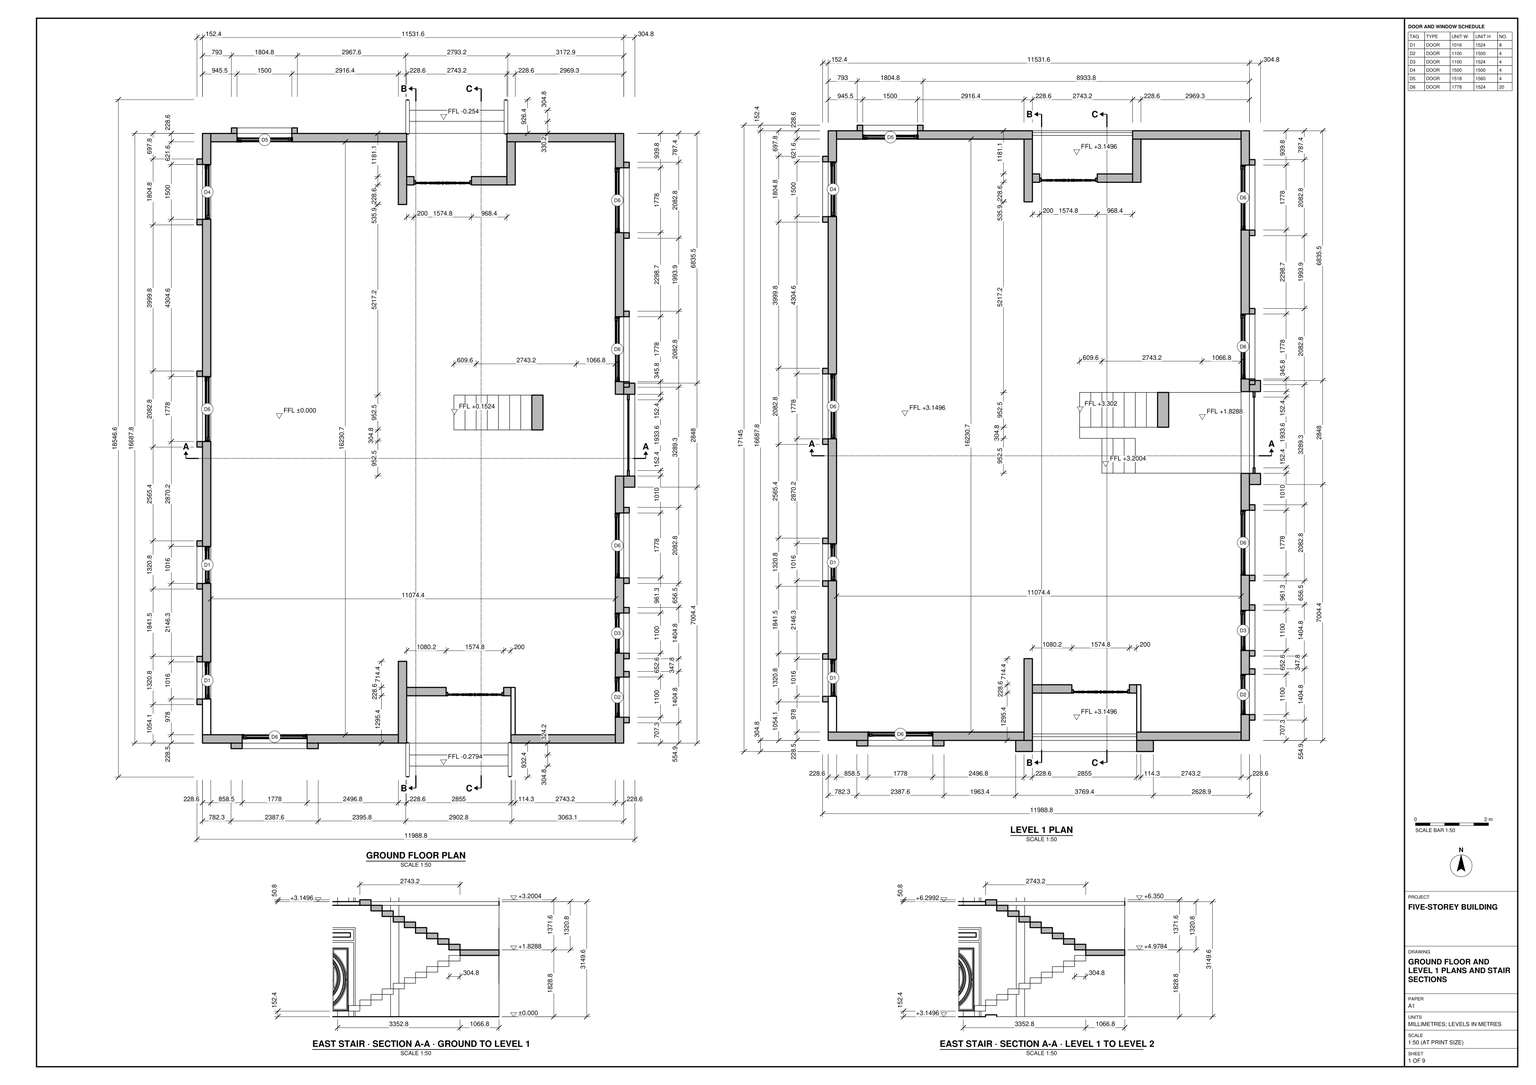
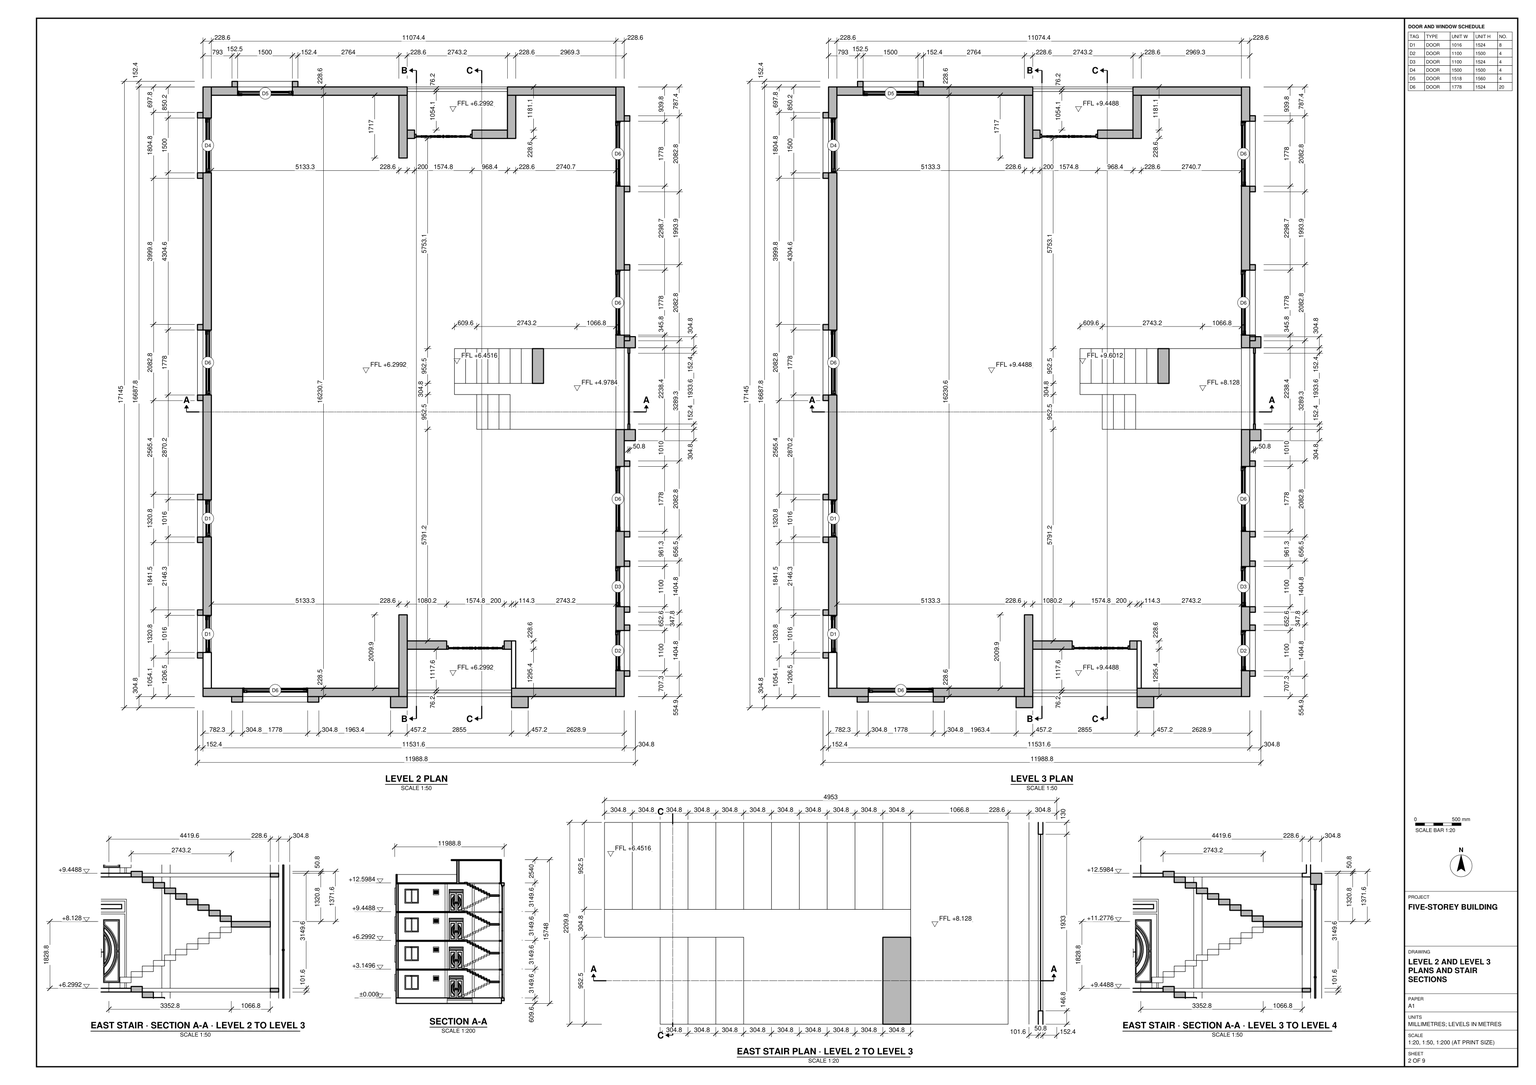
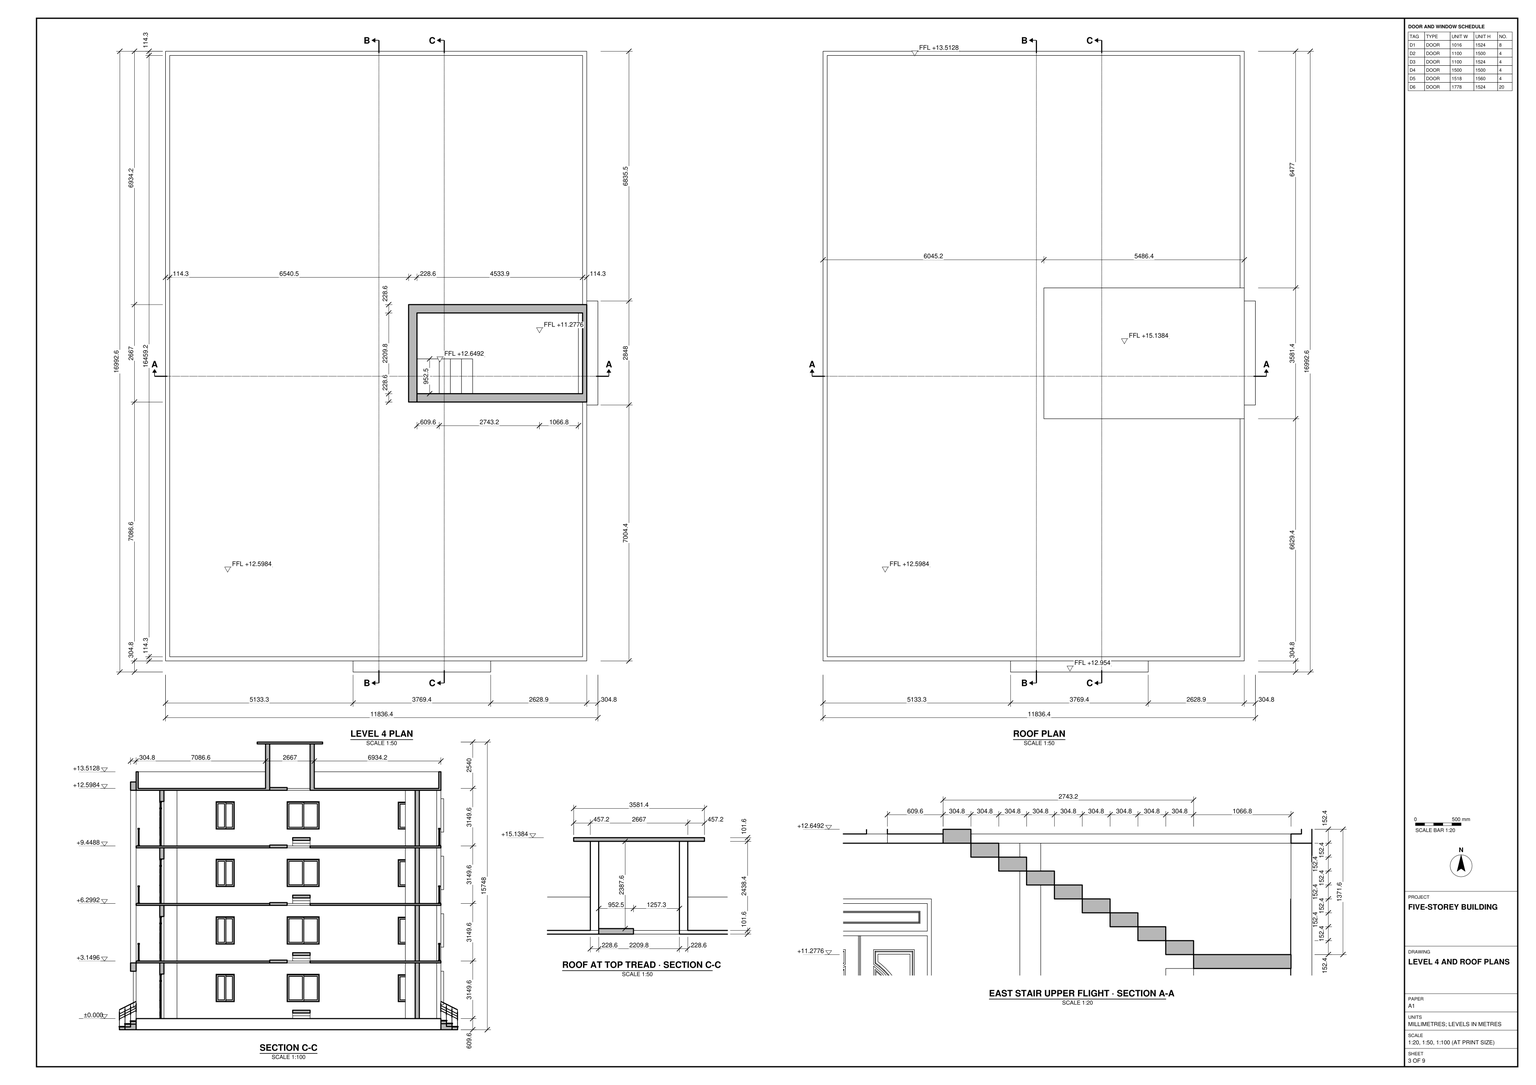
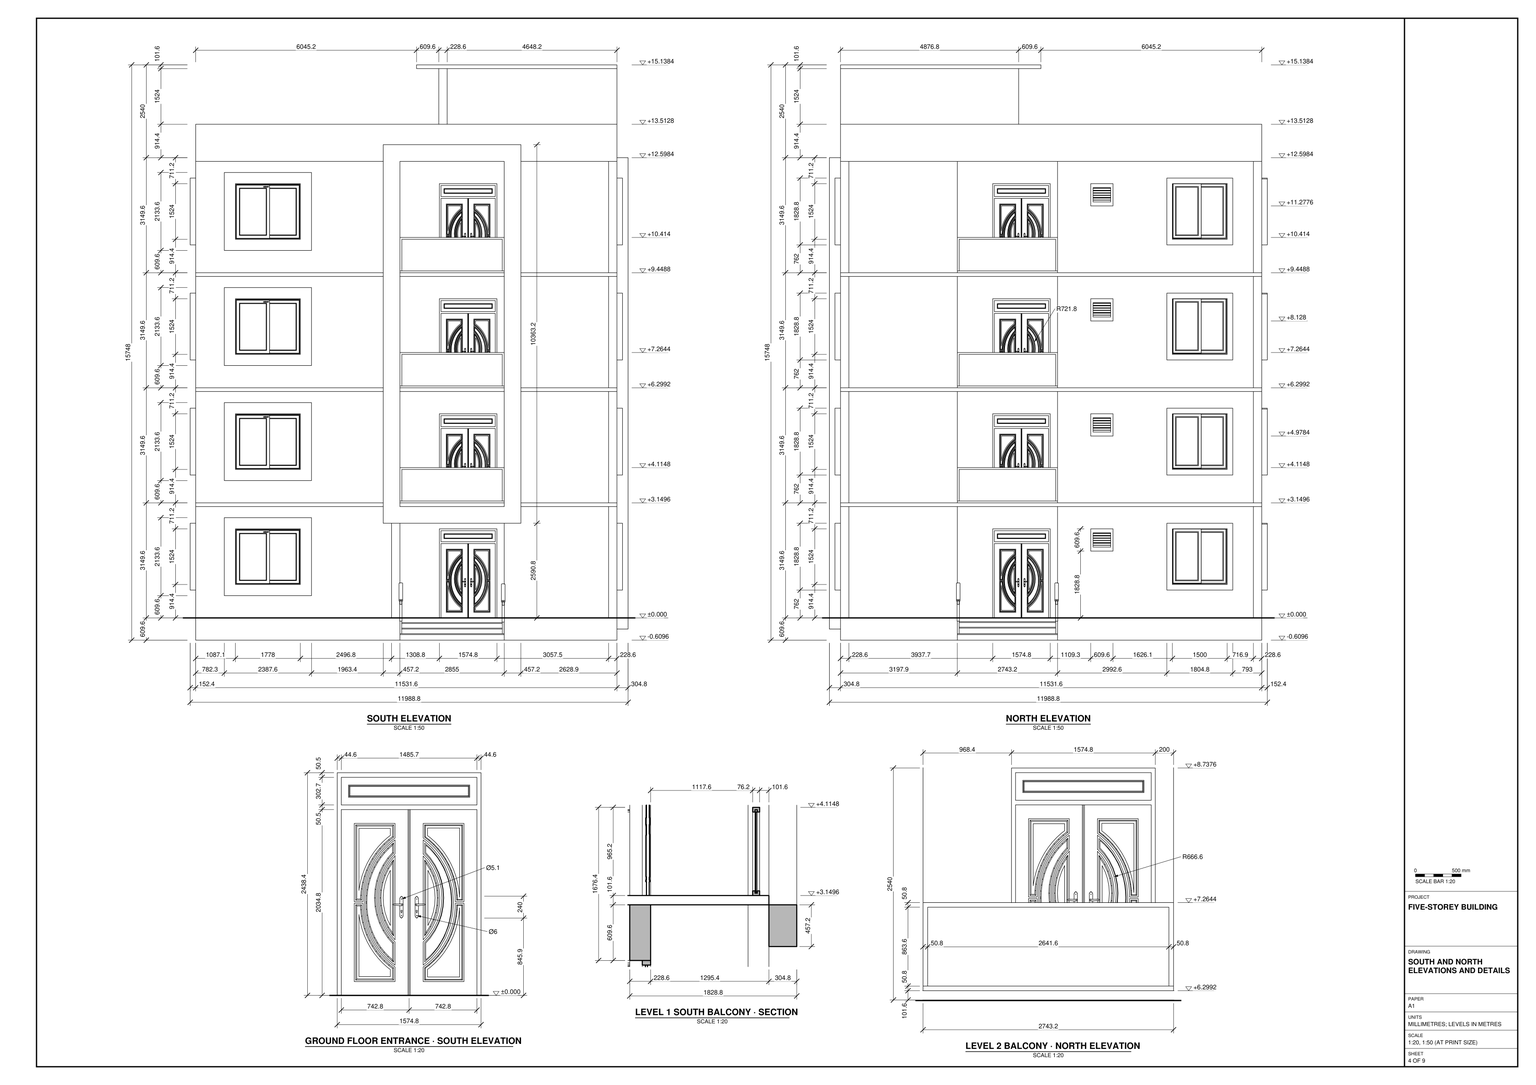
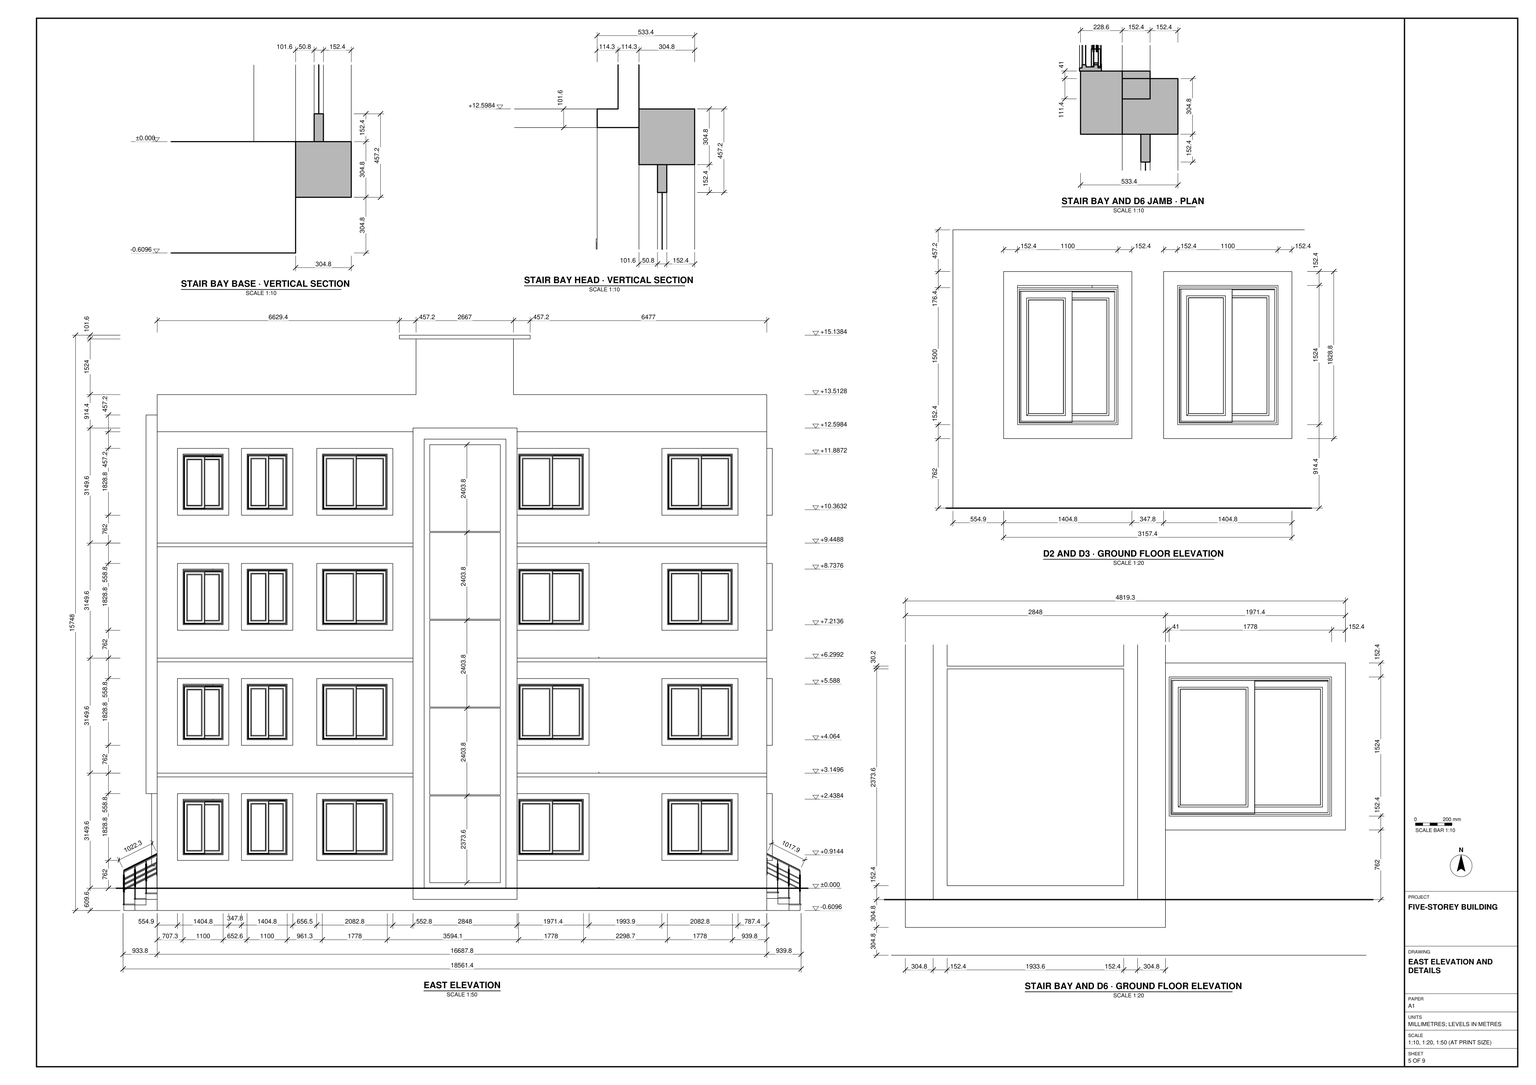
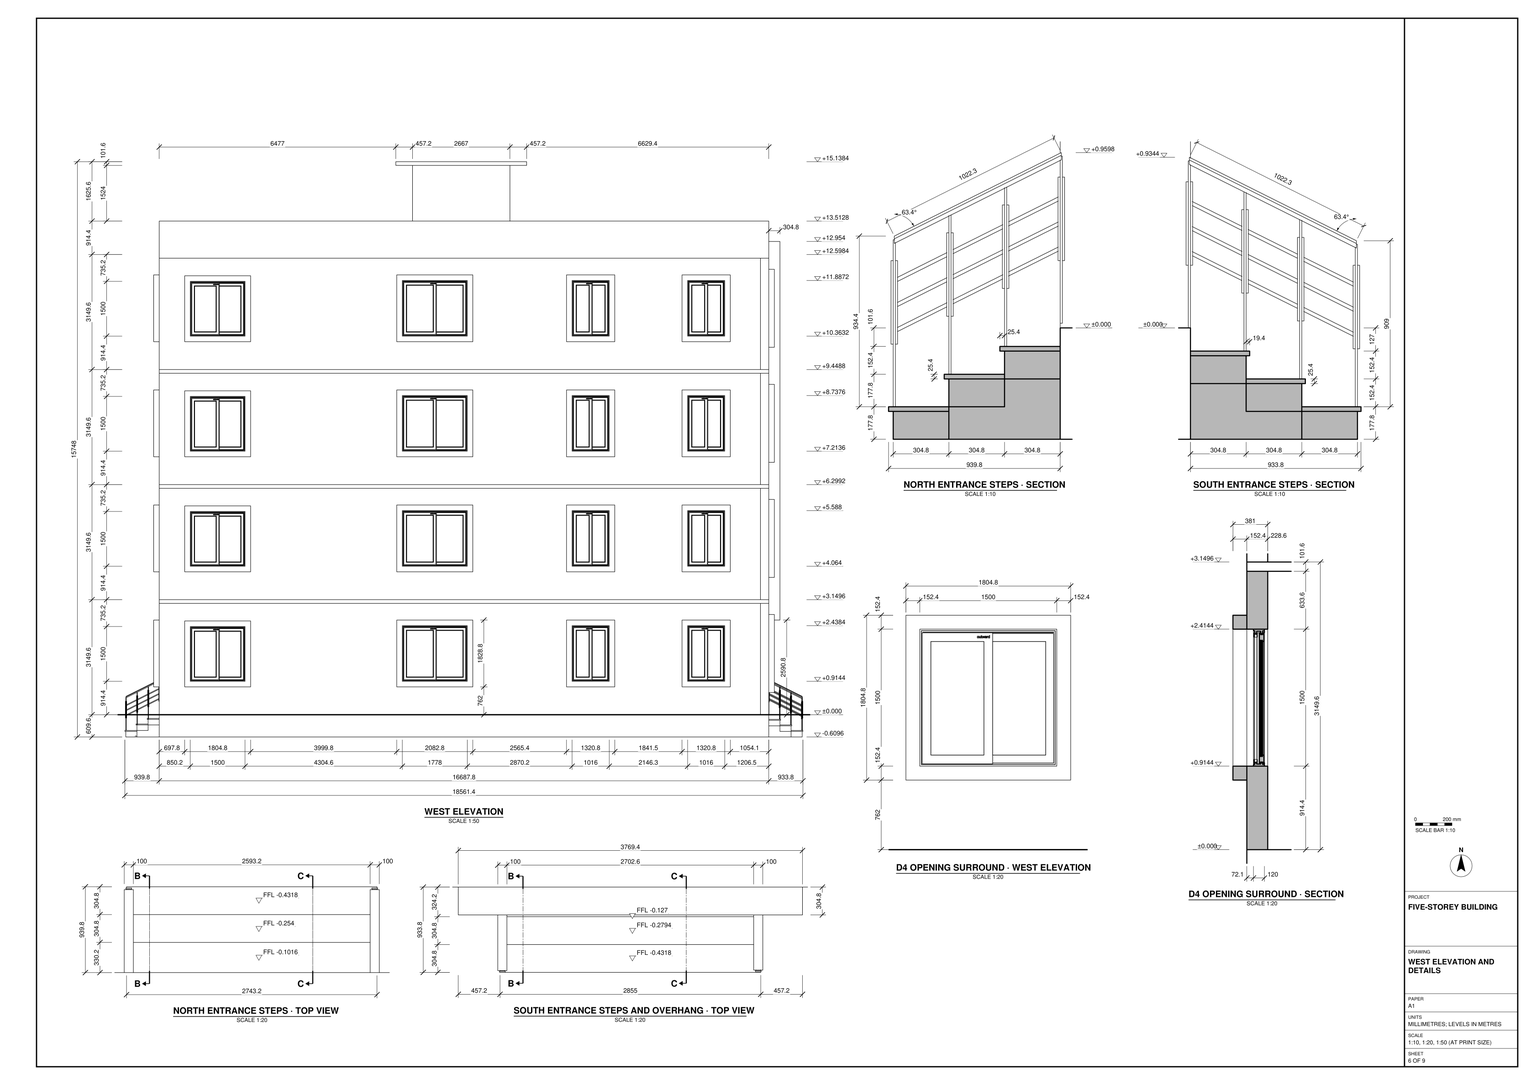
Use task_files/diagram_01.pdf to build the model in SketchUp. Work in millimetres. Set out the building with its short sides facing north and south. The overall extents are 11988.8 mm along X, 18561.4 mm along Y and 15748 mm from base to top. Use finished floor levels of 0 mm, +3149.6 mm, +6299.2 mm, +9448.8 mm and +12598.4 mm relative to the ground floor.

Build the base, floor slabs and perimeter walls, keeping the enclosed floors largely open as shown in plan. Follow the drawn wall thicknesses and reproduce the wall returns that form the recessed entrances at the north and south ends. Include the exterior approach steps and railings. Use the plans and schedule to size and place the doors and window units, retaining the frames and the vertical alignment of corresponding openings.

Use the stair sections to model the two returning flights on the east side, their intermediate landings and the openings through the slabs. At level 4, form the flat roof with its perimeter parapet and the raised enclosure over the stair. Keep shell elements and any furniture or joinery pieces in separate groups or components, and use components for repeated parts. Decor and loose items shown may be any suitable library components. Save one SketchUp model as output_files/five_storey_building_with_east_stair_and_roof_access.skp.

# SketchUp Ruby script. Lengths in millimetres.
U = 1.mm
M = Sketchup.active_model
def pt(a) = Geom::Point3d.new(a.map { |v| v * U })
def face(e, loops, mat)
  f = e.add_face(loops[0].map { |a| pt(a) })
  loops[1..].each { |l| e.add_face(l.map { |a| pt(a) }).erase! }
  f.material = f.back_material = mat if mat
  f
end
# faces: each face lists its corners as indices into pts; further lists are holes
def faces(e, pts, list, mat = nil) = list.each { |f| face(e, (f[0].is_a?(Array) ? f : [f]).map { |l| l.map { |i| pts[i] } }, mat) }
# xy, xz, yz: faces in a plane at the given z, y or x. An outline is a flat list of corners, or four numbers for a rectangle; further outlines are holes
def ring(l) = l.size == 4 ? [[l[0], l[1]], [l[2], l[1]], [l[2], l[3]], [l[0], l[3]]] : l.each_slice(2).to_a
def flat(e, list, mat, &to3) = list.each { |f| face(e, (f[0].is_a?(Array) ? f : [f]).map { |l| ring(l).map { |u, v| to3.(u, v) } }, mat) }
def xy(e, z, list, mat = nil) = flat(e, list, mat) { |x, y| [x, y, z] }
def xz(e, y, list, mat = nil) = flat(e, list, mat) { |x, z| [x, y, z] }
def yz(e, x, list, mat = nil) = flat(e, list, mat) { |y, z| [x, y, z] }
def lines(e, pts, list) = list.each { |a, b| e.add_line(pt(pts[a]), pt(pts[b])) }
# prism: a flat outline (further loops are holes) pulled along v
def prism(e, loops, v, mat = nil)
  f = face(e, loops, mat); d = Geom::Vector3d.new(v.map { |x| x * U })
  f.pushpull(f.normal.samedirection?(d) ? d.length : -d.length)
end
def box(e, o, s, mat = nil) = prism(e, [[o, [o[0] + s[0], o[1], o[2]], [o[0] + s[0], o[1] + s[1], o[2]], [o[0], o[1] + s[1], o[2]]]], [0, 0, s[2]], mat)
def at(x, y, z, deg = 0) = Geom::Transformation.translation(pt([x, y, z])) * Geom::Transformation.rotation(ORIGIN, Z_AXIS, deg.degrees)
def axes(o, x, y, z) = Geom::Transformation.new([*x, 0, *y, 0, *z, 0, *pt(o).to_a, 1])
def part(name) = M.definitions.add(name)
# library, detail: a bought-in or finely detailed component or shape, given as its bounding box
def library(name, o, s) = part(name).tap { |d| box(d.entities, o, s) }
def detail(e, o, s) = box(e.add_group.entities, o, s)
def put(e, d, t, mat = nil) = e.add_instance(d, t).tap { |i| i.material = mat if mat }
def group(e, t, mat = nil) = e.add_group.tap { |g| g.transformation = t; g.material = mat if mat }.entities
root = M.entities
M.materials.add("TEAKcrown-cut").color = [186, 122, 55]
M.materials.add("[Brick Colored Blue]").color = [144, 143, 146]
M.materials.add("[Brick Rough Dark]").color = [94, 77, 53]
M.materials.add("[Color M05]").color = [114, 114, 114]
M.materials.add("[Color M06]").color = [86, 86, 86]
M.materials.add("[Color M07]").color = [58, 58, 58]
M.materials.add("[Translucent Glass Gray]").color = [128, 128, 128]
M.materials["[Translucent Glass Gray]"].alpha = 0.5
M.materials.add("[Translucent Glass Sky Reflection]").color = [124, 138, 181]
M.materials["[Translucent Glass Sky Reflection]"].alpha = 0.5
M.materials.add("[Translucent_Glass_Gray]3").color = [255, 255, 255]
M.materials["[Translucent_Glass_Gray]3"].alpha = 0.5
c1 = part("Component\#10")
box(c1.entities,[0,0,0],[482.6,6.4,94],"[Translucent_Glass_Gray]3")
c2 = part("Ventilation_window")
g1 = group(c2.entities,at(-1953.5,162,0),"TEAKcrown-cut")
xy(g1,-43.2,[[0,0,609.6,76.2]])
xy(g1,63.5,[[63.5,0,546.1,76.2]])
xy(g1,444.5,[[63.5,0,546.1,76.2]])
xy(g1,551.2,[[0,0,609.6,76.2]])
xz(g1,0,[[[0,-43.2,609.6,551.2],[63.5,63.5,546.1,444.5]]],"TEAKcrown-cut")
xz(g1,76.2,[[[0,-43.2,609.6,551.2],[63.5,63.5,546.1,444.5]]])
yz(g1,0,[[0,-43.2,76.2,551.2]])
yz(g1,63.5,[[0,63.5,76.2,63.5,76.2,109.5,0,164.5],[76.2,109.5,76.2,444.5,0,444.5,0,164.5]])
yz(g1,546.1,[[0,63.5,76.2,444.5]])
yz(g1,609.6,[[0,-43.2,76.2,551.2]])
put(g1,c1,axes([63.5,79.8,303.2],[1,0,0],[0,0.58779,0.80902],[0,-0.80902,0.58779]))
put(g1,c1,axes([63.5,80.3,370.9],[1,0,0],[0,0.58779,0.80902],[0,-0.80902,0.58779]))
put(g1,c1,axes([63.5,76.2,109.5],[1,0,0],[0,0.58779,0.80902],[0,-0.80902,0.58779]))
put(g1,c1,axes([63.5,79.8,240.3],[1,0,0],[0,0.58779,0.80902],[0,-0.80902,0.58779]))
put(g1,c1,axes([63.5,76,179.9],[1,0,0],[0,0.58779,0.80902],[0,-0.80902,0.58779]))
c3 = library("AS-120-mm\#4",[0,0,0],[1016,120,1524])
c4 = library("AS-120-mm\#2",[0,0,0],[1500,120,1500])
c5 = library("AS-120-mm\#1",[0,0,0],[1518,120,1560])
c6 = library("AS-120-mm\#3",[0,0,0],[1778,120,1524])
c7 = library("AS-120-mm\#5",[0,0,0],[1778,120,1524])
c8 = library("AS-120-mm\#10",[0,0,0],[1778,120,1524])
c9 = library("AS-120-mm\#7",[0,0,0],[1100,120,1524])
c10 = library("AS-120-mm\#6",[0,0,0],[1100,120,1500])
c11 = library("AS-120-mm\#8",[0,0,0],[1778,120,1524])
c12 = library("AS-120-mm\#9",[0,0,0],[1778,120,1524])
c13 = part("Group\#4")
box(c13.entities,[0,0,0],[2969.3,228.6,3048])
c14 = part("Group\#14")
prism(c14.entities,[[[2743.2,228.6,0],[1774.8,228.6,0],[1774.8,228.6,2438.4],[200,228.6,2438.4],[200,228.6,0],[0,228.6,0],[0,228.6,3048],[2743.2,228.6,3048]]],[0,-228.6,0])
c15 = part("Group\#15")
box(c15.entities,[0,0,0],[228.6,1717,3048])
c16 = part("Group\#8")
box(c16.entities,[0,0,0],[304.8,952.5,152.4])
c17 = part("Group\#10")
box(c17.entities,[0,0,0],[228.6,2238.4,3048])
c18 = part("Group\#6")
box(c18.entities,[0,0,0],[2857.5,228.6,3048])
c19 = part("Group\#7")
box(c19.entities,[0,-1257.3,0],[1066.8,2209.8,152.4])
c20 = part("Group\#2")
prism(c20.entities,[[[228.6,0,0],[228.6,16459.2,0],[228.6,16459.2,3048],[228.6,0,3048]],[[228.6,9804.4,2438.4],[228.6,9804.4,914.4],[228.6,8026.4,914.4],[228.6,8026.4,2438.4]],[[228.6,14109,914.4],[228.6,14109,2414.4],[228.6,15609,2414.4],[228.6,15609,914.4]],[[228.6,977.9,2438.4],[228.6,1993.9,2438.4],[228.6,1993.9,914.4],[228.6,977.9,914.4]],[[228.6,5156.2,2438.4],[228.6,5156.2,914.4],[228.6,4140.2,914.4],[228.6,4140.2,2438.4]]],[-228.6,0,0])
c21 = part("Group\#3")
prism(c21.entities,[[[5361.9,228.6,0],[0,228.6,0],[0,228.6,3048],[5361.9,228.6,3048]],[[2216.9,228.6,914.4],[2216.9,228.6,2438.4],[716.8,228.6,2438.4],[716.8,228.6,914.4]],[[3843,228.6,1828.8],[4452.6,228.6,1828.8],[4452.6,228.6,2438.4],[3843,228.6,2438.4]]],[0,-228.6,0])
c22 = part("Group\#11")
prism(c22.entities,[[[0,0,0],[1080.2,0,0],[1080.2,0,2438.4],[2655,0,2438.4],[2655,0,0],[2855,0,0],[2855,0,3048],[0,0,3048]]],[0,228.6,0])
c23 = library("Group\#55",[0,0,0],[2120,123.6,2900])
c24 = part("Group\#12")
box(c24.entities,[0,0,0],[114.3,1295.4,3048])
c25 = part("Group\#13")
box(c25.entities,[0,0,0],[228.6,1181.1,3048])
c26 = part("Group\#1")
prism(c26.entities,[[[5361.9,228.6,0],[0,228.6,0],[0,228.6,3048],[5361.9,228.6,3048]],[[2865.1,228.6,2438.4],[1087.1,228.6,2438.4],[1087.1,228.6,914.4],[2865.1,228.6,914.4]]],[0,-228.6,0])
c27 = part("Group\#35")
prism(c27.entities,[[[0,16687.8,0],[11531.6,16687.8,0],[11531.6,0,0],[0,0,0]],[[6883.4,9525,0],[6883.4,8267.7,0],[7493,8267.7,0],[7493,7315.2,0],[11303,7315.2,0],[11303,9525,0]]],[0,0,101.6])
c28 = part("Group\#21")
g2 = group(c28.entities,at(0,1.6,0))
prism(g2,[[[0,76.2,0],[0,0,0],[0,0,50.8],[0,25.4,50.8],[0,25.4,25.4],[0,50.8,25.4],[0,50.8,50.8],[0,76.2,50.8]]],[2743.2,0,0])
g3 = group(c28.entities,at(0,1.6,965.2))
xy(g3,-914.4,[[0,0,50.8,25.4],[2692.4,0,2743.2,25.4],[0,50.8,50.8,76.2],[2692.4,50.8,2743.2,76.2]])
xy(g3,-50.8,[[50.8,0,2692.4,25.4],[50.8,25.4,2692.4,50.8],[50.8,50.8,2692.4,76.2]])
xy(g3,-25.4,[[0,25.4,2743.2,50.8]])
xy(g3,0,[[0,0,2743.2,76.2]])
xz(g3,0,[[0,-914.4,0,0,2743.2,0,2743.2,-914.4,2692.4,-914.4,2692.4,-50.8,50.8,-50.8,50.8,-914.4]])
xz(g3,25.4,[[0,-914.4,50.8,-914.4,50.8,-50.8,2692.4,-50.8,2692.4,-914.4,2743.2,-914.4,2743.2,-25.4,0,-25.4]])
xz(g3,50.8,[[0,-914.4,0,-25.4,2743.2,-25.4,2743.2,-914.4,2692.4,-914.4,2692.4,-50.8,50.8,-50.8,50.8,-914.4]])
xz(g3,76.2,[[0,-914.4,50.8,-914.4,50.8,-50.8,2692.4,-50.8,2692.4,-914.4,2743.2,-914.4,2743.2,0,0,0]])
yz(g3,0,[[0,-914.4,25.4,-914.4,25.4,-25.4,50.8,-25.4,50.8,-914.4,76.2,-914.4,76.2,0,0,0]])
yz(g3,50.8,[[0,-914.4,25.4,-50.8],[50.8,-914.4,76.2,-50.8]])
yz(g3,2692.4,[[0,-914.4,25.4,-50.8],[50.8,-914.4,76.2,-50.8]])
yz(g3,2743.2,[[0,-914.4,0,0,76.2,0,76.2,-914.4,50.8,-914.4,50.8,-25.4,25.4,-25.4,25.4,-914.4]])
p = [[2692.4,0,-50.8],[2692.4,-1.6,-50.8]]
lines(g3,p,[[0,1]])
g4 = group(c28.entities,at(0,39.7,25.4),"[Translucent Glass Sky Reflection]")
box(g4,[0,0,0],[2743.2,10.2,889])
c29 = part("Group\#23")
prism(c29.entities,[[[0,152.4,0],[0,152.4,2133.6],[2387.6,152.4,2133.6],[2387.6,152.4,0]],[[2082.8,152.4,304.8],[2082.8,152.4,1828.8],[304.8,152.4,1828.8],[304.8,152.4,304.8]]],[0,-152.4,0])
c30 = part("Group\#24")
prism(c30.entities,[[[0,0,0],[0,0,1828.8],[0,1320.8,1828.8],[0,1320.8,0]],[[0,1168.4,1676.4],[0,152.4,1676.4],[0,152.4,152.4],[0,1168.4,152.4]]],[152.4,0,0])
c31 = part("Group\#25")
prism(c31.entities,[[[152.4,0,1828.8],[152.4,0,0],[152.4,2082.8,0],[152.4,2082.8,1828.8]],[[152.4,1930.4,1676.4],[152.4,1930.4,152.4],[152.4,152.4,152.4],[152.4,152.4,1676.4]]],[-152.4,0,0])
c32 = part("Group\#26")
prism(c32.entities,[[[0,0,1804.8],[0,1804.8,1804.8],[0,1804.8,0],[0,0,0]],[[0,1652.4,1652.4],[0,152.4,1652.4],[0,152.4,152.4],[0,1652.4,152.4]]],[152.4,0,0])
c33 = part("Group\#27")
prism(c33.entities,[[[1804.8,152.4,1828.8],[1804.8,152.4,0],[0,152.4,0],[0,152.4,1828.8]],[[1652.4,152.4,152.4],[1652.4,152.4,1676.4],[152.4,152.4,1676.4],[152.4,152.4,152.4]]],[0,-152.4,0])
c34 = part("Group139\#2")
xy(c34.entities,0,[[-966.8,-5994.4,966.8,-3620.8],[-966.8,-3590.6,966.8,-1217],[-966.8,-1186.8,966.8,1186.8],[-966.8,1217,966.8,3590.6],[-966.8,3620.8,966.8,5994.4]])
c35 = part("Group138\#1")
prism(c35.entities,[[[-1119.2,6146.8,0],[1119.2,6146.8,0],[1119.2,-6146.8,0],[-1119.2,-6146.8,0]],[[966.8,3620.8,0],[966.8,5994.4,0],[-966.8,5994.4,0],[-966.8,3620.8,0]],[[-966.8,1217,0],[966.8,1217,0],[966.8,3590.6,0],[-966.8,3590.6,0]],[[-966.8,-1186.8,0],[966.8,-1186.8,0],[966.8,1186.8,0],[-966.8,1186.8,0]],[[966.8,-3590.6,0],[966.8,-1217,0],[-966.8,-1217,0],[-966.8,-3590.6,0]],[[-966.8,-5994.4,0],[966.8,-5994.4,0],[966.8,-3620.8,0],[-966.8,-3620.8,0]]],[0,0,50.8])
put(c35.entities,c34,at(0,0,25.4),"[Translucent Glass Gray]")
c36 = library("Group\#43",[25,-6,-25.4],[2793.2,950.4,1569.4])
c37 = part("Group\#44")
box(c37.entities,[0,0,0],[2855,304.8,152.4])
c38 = library("Group\#47",[0,0,0],[100,950.4,1391.6])
c39 = library("Group\#49",[0,0,0],[100,950.4,1391.6])
c40 = part("Group\#50")
box(c40.entities,[0,0,0],[2854.6,324.2,25.4])
c41 = part("Group\#51")
box(c41.entities,[0,0,0],[2743.2,330.2,25.4])
c42 = part("Group\#52")
prism(c42.entities,[[[152.4,2082.8,0],[152.4,2082.8,1828.8],[152.4,0,1828.8],[152.4,0,0]],[[152.4,152.4,152.4],[152.4,152.4,1676.4],[152.4,1930.4,1676.4],[152.4,1930.4,152.4]]],[-152.4,0,0])
c43 = part("Group\#53")
prism(c43.entities,[[[0,0,0],[0,0,1828.8],[0,1404.8,1828.8],[0,1404.8,0]],[[0,152.4,1676.4],[0,152.4,152.4],[0,1252.4,152.4],[0,1252.4,1676.4]]],[152.4,0,0])
put(root,c2,axes([6177.5,17342.5,1873.1],[1,0,0],[0,0.9306,0],[0,0,1.02564]))
put(root,c2,axes([6177.5,17342.5,5022.7],[1,0,0],[0,0.9306,0],[0,0,1.02564]))
put(root,c2,axes([6177.5,17342.5,8172.3],[1,0,0],[0,0.9306,0],[0,0,1.02564]))
put(root,c2,axes([6177.5,17342.5,11321.9],[1,0,0],[0,0.9306,0],[0,0,1.02564]))
g5 = group(root,at(152.4,933.8,-152.4))
box(g5,[0,0,-457.2],[11531.6,16687.8,609.6])
g6 = group(root,at(152.4,933.8,0))
p = [[13804.3,12092.4,35.2],[13804.3,12092.4,0]]
lines(g6,p,[[0,1]])
put(g6,c3,at(72.1,5384.8,914.4,-90))
put(g6,c4,at(72.1,15837.6,914.4,-90))
put(g6,c5,at(945.4,16453.5,914.4))
put(g6,c6,at(72.1,10033,914.4,-90))
put(g6,c7,at(11297.3,15748,914.4,-90))
put(g6,c8,at(1087.1,114.3,914.4))
put(g6,c3,at(72.1,2222.5,914.4,-90))
put(g6,c9,at(11297.3,3559.9,914.4,-90))
put(g6,c10,at(11297.3,1807.3,914.4,-90))
put(g6,c11,at(11297.3,6299.2,914.4,-90))
put(g6,c12,at(11297.3,11671.3,914.4,-90))
put(g6,c13,at(8333.7,16459.2,0))
put(g6,c14,at(5590.5,15278.1,0))
put(g6,c15,at(5361.9,14742.2,0))
put(g6,c16,at(7188.2,8572.5,152.4))
put(g6,c16,at(8102.6,8572.5,609.6))
put(g6,c17,at(5361.9,0,0))
put(g6,c18,at(8445.5,0,0))
put(g6,c16,at(9626.6,7315.2,1981.2))
g7 = group(g6,at(11303,0,0))
prism(g7,[[[228.6,16687.8,3048],[228.6,9547.5,3048],[228.6,9547.5,0],[228.6,16687.8,0]],[[228.6,13970,914.4],[228.6,13970,2438.4],[228.6,15748,2438.4],[228.6,15748,914.4]],[[228.6,11671.3,2438.4],[228.6,11671.3,914.4],[228.6,9893.3,914.4],[228.6,9893.3,2438.4]]],[-228.6,0,0])
prism(g7,[[[228.6,0,0],[228.6,7309.2,0],[228.6,7309.2,3048],[228.6,0,3048]],[[228.6,4521.2,2438.4],[228.6,6299.2,2438.4],[228.6,6299.2,914.4],[228.6,4521.2,914.4]],[[228.6,2459.9,914.4],[228.6,2459.9,2438.4],[228.6,3559.9,2438.4],[228.6,3559.9,914.4]],[[228.6,707.3,2438.4],[228.6,1807.3,2438.4],[228.6,1807.3,914.4],[228.6,707.3,914.4]]],[-228.6,0,0])
p = [[0,9547.5,3048],[0,7309.2,3048]]
lines(g7,p,[[0,1]])
put(g6,c16,at(7493,8572.5,304.8))
put(g6,c19,at(10236.2,8572.5,1676.4))
put(g6,c16,at(7797.8,8572.5,457.2))
put(g6,c16,at(6883.4,8572.5,0))
put(g6,c20,at(0,228.6,0))
put(g6,c16,at(8407.4,7315.2,2590.8))
put(g6,c16,at(9017,7315.2,2286))
put(g6,c16,at(8712.2,8572.5,914.4))
put(g6,c21,at(228.6,16459.2,0))
put(g6,c16,at(8407.4,8572.5,762))
put(g6,c16,at(9626.6,8572.5,1371.6))
put(g6,c16,at(9931.4,8572.5,1524))
put(g6,c22,at(5590.5,1295.4,0))
put(g6,c23,axes([8245.5,1386.6,0],[-0.74283,0,0],[0,-0.76,0],[0,0,0.84083]))
put(g6,c24,at(8445.5,228.6,0))
put(g6,c16,at(9321.8,7315.2,2133.6))
put(g6,c16,at(9321.8,8572.5,1219.2))
put(g6,c16,at(9017,8572.5,1066.8))
put(g6,c16,at(8102.6,7315.2,2743.2))
put(g6,c16,at(8712.2,7315.2,2438.4))
put(g6,c16,at(7797.8,7315.2,2895.6))
put(g6,c16,at(9931.4,7315.2,1828.8))
put(g6,c16,at(7493,7315.2,3048))
put(g6,c25,at(8333.7,15278.1,0))
put(g6,c26,at(0,0,0))
put(g6,c27,at(0,0,3048))
put(g6,c23,axes([7365.3,15392.4,0],[-0.74283,0,0],[0,-0.76,0],[0,0,0.84083]))
g8 = group(root,at(152.4,933.8,3149.6))
p = [[13804.3,12092.4,35.2],[13804.3,12092.4,0]]
lines(g8,p,[[0,1]])
put(g8,c3,at(72.1,5384.8,914.4,-90))
put(g8,c4,at(72.1,15837.6,914.4,-90))
put(g8,c5,at(945.4,16453.5,914.4))
put(g8,c6,at(72.1,10033,914.4,-90))
put(g8,c7,at(11297.3,15748,914.4,-90))
put(g8,c8,at(1087.1,114.3,914.4))
put(g8,c3,at(72.1,2222.5,914.4,-90))
put(g8,c9,at(11297.3,3559.9,914.4,-90))
put(g8,c10,at(11297.3,1807.3,914.4,-90))
put(g8,c11,at(11297.3,6299.2,914.4,-90))
put(g8,c12,at(11297.3,11671.3,914.4,-90))
put(g8,c13,at(8333.7,16459.2,0))
put(g8,c14,at(5590.5,15278.1,0))
put(g8,c15,at(5361.9,14742.2,0))
put(g8,c16,at(7188.2,8572.5,152.4))
put(g8,c16,at(8102.6,8572.5,609.6))
put(g8,c17,at(5361.9,0,0))
put(g8,c18,at(8445.5,0,0))
put(g8,c16,at(9626.6,7315.2,1981.2))
g9 = group(g8,at(11303,0,0))
prism(g9,[[[0,16687.8,0],[0,9547.5,0],[0,9547.5,3048],[0,16687.8,3048]],[[0,11671.3,914.4],[0,11671.3,2438.4],[0,9893.3,2438.4],[0,9893.3,914.4]],[[0,13970,2438.4],[0,13970,914.4],[0,15748,914.4],[0,15748,2438.4]]],[228.6,0,0])
prism(g9,[[[228.6,0,0],[228.6,7309.2,0],[228.6,7309.2,3048],[228.6,0,3048]],[[228.6,4521.2,2438.4],[228.6,6299.2,2438.4],[228.6,6299.2,914.4],[228.6,4521.2,914.4]],[[228.6,2459.9,914.4],[228.6,2459.9,2438.4],[228.6,3559.9,2438.4],[228.6,3559.9,914.4]],[[228.6,707.3,2438.4],[228.6,1807.3,2438.4],[228.6,1807.3,914.4],[228.6,707.3,914.4]]],[-228.6,0,0])
put(g8,c16,at(7493,8572.5,304.8))
put(g8,c19,at(10236.2,8572.5,1676.4))
put(g8,c16,at(7797.8,8572.5,457.2))
put(g8,c16,at(6883.4,8572.5,0))
put(g8,c20,at(0,228.6,0))
put(g8,c16,at(8407.4,7315.2,2590.8))
put(g8,c16,at(9017,7315.2,2286))
put(g8,c16,at(8712.2,8572.5,914.4))
put(g8,c21,at(228.6,16459.2,0))
put(g8,c16,at(8407.4,8572.5,762))
put(g8,c16,at(9626.6,8572.5,1371.6))
put(g8,c16,at(9931.4,8572.5,1524))
put(g8,c22,at(5590.5,1295.4,0))
put(g8,c23,axes([8245.5,1386.6,0],[-0.74283,0,0],[0,-0.76,0],[0,0,0.84083]))
put(g8,c24,at(8445.5,228.6,0))
put(g8,c16,at(9321.8,7315.2,2133.6))
put(g8,c16,at(9321.8,8572.5,1219.2))
put(g8,c16,at(9017,8572.5,1066.8))
put(g8,c16,at(8102.6,7315.2,2743.2))
put(g8,c16,at(8712.2,7315.2,2438.4))
put(g8,c16,at(7797.8,7315.2,2895.6))
put(g8,c16,at(9931.4,7315.2,1828.8))
put(g8,c16,at(7493,7315.2,3048))
put(g8,c25,at(8333.7,15278.1,0))
put(g8,c26,at(0,0,0))
put(g8,c27,at(0,0,3048))
put(g8,c23,axes([7365.3,15392.4,0],[-0.74283,0,0],[0,-0.76,0],[0,0,0.84083]))
g10 = group(root,at(152.4,933.8,6299.2))
p = [[13804.3,12092.4,35.2],[13804.3,12092.4,0]]
lines(g10,p,[[0,1]])
put(g10,c3,at(72.1,5384.8,914.4,-90))
put(g10,c4,at(72.1,15837.6,914.4,-90))
put(g10,c5,at(945.4,16453.5,914.4))
put(g10,c6,at(72.1,10033,914.4,-90))
put(g10,c7,at(11297.3,15748,914.4,-90))
put(g10,c8,at(1087.1,114.3,914.4))
put(g10,c3,at(72.1,2222.5,914.4,-90))
put(g10,c9,at(11297.3,3559.9,914.4,-90))
put(g10,c10,at(11297.3,1807.3,914.4,-90))
put(g10,c11,at(11297.3,6299.2,914.4,-90))
put(g10,c12,at(11297.3,11671.3,914.4,-90))
put(g10,c13,at(8333.7,16459.2,0))
put(g10,c14,at(5590.5,15278.1,0))
put(g10,c15,at(5361.9,14742.2,0))
put(g10,c16,at(7188.2,8572.5,152.4))
put(g10,c16,at(8102.6,8572.5,609.6))
put(g10,c17,at(5361.9,0,0))
put(g10,c18,at(8445.5,0,0))
put(g10,c16,at(9626.6,7315.2,1981.2))
g11 = group(g10,at(11303,0,0))
prism(g11,[[[0,16687.8,0],[0,9547.5,0],[0,9547.5,3048],[0,16687.8,3048]],[[0,13970,2438.4],[0,13970,914.4],[0,15748,914.4],[0,15748,2438.4]],[[0,11671.3,914.4],[0,11671.3,2438.4],[0,9893.3,2438.4],[0,9893.3,914.4]]],[228.6,0,0])
prism(g11,[[[228.6,0,0],[228.6,7309.2,0],[228.6,7309.2,3048],[228.6,0,3048]],[[228.6,4521.2,2438.4],[228.6,6299.2,2438.4],[228.6,6299.2,914.4],[228.6,4521.2,914.4]],[[228.6,2459.9,914.4],[228.6,2459.9,2438.4],[228.6,3559.9,2438.4],[228.6,3559.9,914.4]],[[228.6,707.3,2438.4],[228.6,1807.3,2438.4],[228.6,1807.3,914.4],[228.6,707.3,914.4]]],[-228.6,0,0])
put(g10,c16,at(7493,8572.5,304.8))
put(g10,c19,at(10236.2,8572.5,1676.4))
put(g10,c16,at(7797.8,8572.5,457.2))
put(g10,c16,at(6883.4,8572.5,0))
put(g10,c20,at(0,228.6,0))
put(g10,c16,at(8407.4,7315.2,2590.8))
put(g10,c16,at(9017,7315.2,2286))
put(g10,c16,at(8712.2,8572.5,914.4))
put(g10,c21,at(228.6,16459.2,0))
put(g10,c16,at(8407.4,8572.5,762))
put(g10,c16,at(9626.6,8572.5,1371.6))
put(g10,c16,at(9931.4,8572.5,1524))
put(g10,c22,at(5590.5,1295.4,0))
put(g10,c23,axes([8245.5,1386.6,0],[-0.74283,0,0],[0,-0.76,0],[0,0,0.84083]))
put(g10,c24,at(8445.5,228.6,0))
put(g10,c16,at(9321.8,7315.2,2133.6))
put(g10,c16,at(9321.8,8572.5,1219.2))
put(g10,c16,at(9017,8572.5,1066.8))
put(g10,c16,at(8102.6,7315.2,2743.2))
put(g10,c16,at(8712.2,7315.2,2438.4))
put(g10,c16,at(7797.8,7315.2,2895.6))
put(g10,c16,at(9931.4,7315.2,1828.8))
put(g10,c16,at(7493,7315.2,3048))
put(g10,c25,at(8333.7,15278.1,0))
put(g10,c26,at(0,0,0))
put(g10,c27,at(0,0,3048))
put(g10,c23,axes([7365.3,15392.4,0],[-0.74283,0,0],[0,-0.76,0],[0,0,0.84083]))
put(root,c28,at(5742.9,17493,9448.8))
put(root,c28,at(5742.9,17493,6299.2))
put(root,c28,at(5742.9,17493,3149.6))
put(root,c28,axes([5742.9,1033.8,9448.8],[1.04077,0,0],[0,1,0],[0,0,1]))
put(root,c28,axes([5742.9,1033.8,6299.2],[1.04077,0,0],[0,1,0],[0,0,1]))
put(root,c28,axes([5742.9,1033.8,3149.6],[1.04077,0,0],[0,1,0],[0,0,1]))
g12 = group(root,at(5285.7,629,2590.8),"[Color M07]")
prism(g12,[[[3769.4,0,0],[3769.4,0,10363.2],[0,0,10363.2],[0,0,0]],[[457.2,0,457.2],[457.2,0,9906],[3312.2,0,9906],[3312.2,0,457.2]]],[0,304.8,0])
put(root,c29,at(934.7,781.4,10058.4),"[Color M07]")
put(root,c29,at(934.7,781.4,6908.8),"[Color M07]")
put(root,c29,at(934.7,781.4,3759.2),"[Color M07]")
put(root,c29,at(934.7,781.4,609.6),"[Color M07]")
put(root,c30,at(0,1987.9,7061.2),"[Color M05]")
put(root,c30,at(0,1987.9,3911.6),"[Color M05]")
put(root,c30,at(0,1987.9,762),"[Color M05]")
put(root,c30,at(0,5150.2,762),"[Color M05]")
put(root,c30,at(0,5150.2,3911.6),"[Color M05]")
put(root,c30,at(0,5150.2,7061.2),"[Color M05]")
put(root,c30,at(0,5150.2,10210.8),"[Color M05]")
put(root,c31,at(0,9036.4,10210.8),"[Color M05]")
put(root,c31,at(0,9036.4,7061.2),"[Color M05]")
put(root,c31,at(0,9036.4,3911.6),"[Color M05]")
put(root,c31,at(0,9036.4,762),"[Color M05]")
put(root,c32,at(0,15119,762),"[Color M05]")
put(root,c32,at(0,15119,3911.6),"[Color M05]")
put(root,c32,at(0,15119,7061.2),"[Color M05]")
put(root,c33,at(945.4,17621.6,10210.8),"[Color M05]")
put(root,c33,at(945.4,17621.6,7061.2),"[Color M05]")
put(root,c33,at(945.5,17621.6,3911.6),"[Color M05]")
put(root,c33,at(945.5,17621.6,762),"[Color M05]")
put(root,c32,at(0,15119,10210.8),"[Color M05]")
put(root,c30,at(0,1987.9,10210.8),"[Color M05]")
g13 = group(root,at(152.4,933.8,9448.8))
p = [[13804.3,12092.4,35.2],[13804.3,12092.4,0]]
lines(g13,p,[[0,1]])
put(g13,c3,at(72.1,5384.8,914.4,-90))
put(g13,c4,at(72.1,15837.6,914.4,-90))
put(g13,c5,at(945.4,16453.5,914.4))
put(g13,c6,at(72.1,10033,914.4,-90))
put(g13,c7,at(11297.3,15748,914.4,-90))
put(g13,c8,at(1087.1,114.3,914.4))
put(g13,c3,at(72.1,2222.5,914.4,-90))
put(g13,c9,at(11297.3,3559.9,914.4,-90))
put(g13,c10,at(11297.3,1807.3,914.4,-90))
put(g13,c11,at(11297.3,6299.2,914.4,-90))
put(g13,c12,at(11297.3,11671.3,914.4,-90))
put(g13,c13,at(8333.7,16459.2,0))
put(g13,c14,at(5590.5,15278.1,0))
put(g13,c15,at(5361.9,14742.2,0))
put(g13,c16,at(7188.2,8572.5,152.4))
put(g13,c16,at(8102.6,8572.5,609.6))
put(g13,c17,at(5361.9,0,0))
put(g13,c18,at(8445.5,0,0))
put(g13,c16,at(9626.6,7315.2,1981.2))
g14 = group(g13,at(11303,0,0))
prism(g14,[[[228.6,16687.8,3048],[228.6,9547.5,3048],[228.6,9547.5,0],[228.6,16687.8,0]],[[228.6,11671.3,2438.4],[228.6,11671.3,914.4],[228.6,9893.3,914.4],[228.6,9893.3,2438.4]],[[228.6,13970,914.4],[228.6,13970,2438.4],[228.6,15748,2438.4],[228.6,15748,914.4]]],[-228.6,0,0])
prism(g14,[[[228.6,0,0],[228.6,7309.2,0],[228.6,7309.2,3048],[228.6,0,3048]],[[228.6,4521.2,2438.4],[228.6,6299.2,2438.4],[228.6,6299.2,914.4],[228.6,4521.2,914.4]],[[228.6,2459.9,914.4],[228.6,2459.9,2438.4],[228.6,3559.9,2438.4],[228.6,3559.9,914.4]],[[228.6,707.3,2438.4],[228.6,1807.3,2438.4],[228.6,1807.3,914.4],[228.6,707.3,914.4]]],[-228.6,0,0])
p = [[0,9547.5,3048],[0,7309.2,3048]]
lines(g14,p,[[0,1]])
put(g13,c16,at(7493,8572.5,304.8))
put(g13,c19,at(10236.2,8572.5,1676.4))
put(g13,c16,at(7797.8,8572.5,457.2))
put(g13,c16,at(6883.4,8572.5,0))
put(g13,c20,at(0,228.6,0))
put(g13,c16,at(8407.4,7315.2,2590.8))
put(g13,c16,at(9017,7315.2,2286))
put(g13,c16,at(8712.2,8572.5,914.4))
put(g13,c21,at(228.6,16459.2,0))
put(g13,c16,at(8407.4,8572.5,762))
put(g13,c16,at(9626.6,8572.5,1371.6))
put(g13,c16,at(9931.4,8572.5,1524))
put(g13,c22,at(5590.5,1295.4,0))
put(g13,c23,axes([8245.5,1386.6,0],[-0.74283,0,0],[0,-0.76,0],[0,0,0.84083]))
put(g13,c24,at(8445.5,228.6,0))
put(g13,c16,at(9321.8,7315.2,2133.6))
put(g13,c16,at(9321.8,8572.5,1219.2))
put(g13,c16,at(9017,8572.5,1066.8))
put(g13,c16,at(8102.6,7315.2,2743.2))
put(g13,c16,at(8712.2,7315.2,2438.4))
put(g13,c16,at(7797.8,7315.2,2895.6))
put(g13,c16,at(9931.4,7315.2,1828.8))
put(g13,c16,at(7493,7315.2,3048))
put(g13,c25,at(8333.7,15278.1,0))
put(g13,c26,at(0,0,0))
g15 = group(g13,at(0,0,3048))
xy(g15,0,[[[0,0,11531.6,16687.8],[7493,7315.2,11303,7315.2,11303,9525,6883.4,9525,6883.4,8267.7,7493,8267.7]]])
xy(g15,101.6,[[114.3,114.3,11417.3,114.3,11417.3,7086.6,6654.8,7086.6,6654.8,9753.6,11417.3,9753.6,11417.3,16573.5,114.3,16573.5],[6883.4,7315.2,7493,8267.7],[11303,7315.2,11417.3,9525]])
xy(g15,1016,[[0,0,11531.6,0,11531.6,7086.6,11417.3,7086.6,11417.3,114.3,114.3,114.3,114.3,16573.5,11417.3,16573.5,11417.3,9753.6,11531.6,9753.6,11531.6,16687.8,0,16687.8]])
xy(g15,2540,[[6654.8,7086.6,6883.4,7086.6,6883.4,9525,11531.6,9525,11531.6,9753.6,6654.8,9753.6],[6883.4,7086.6,11531.6,7086.6,11531.6,9525,11417.3,9525,11417.3,7315.2,6883.4,7315.2]])
xz(g15,0,[[0,0,11531.6,1016]])
xz(g15,114.3,[[114.3,101.6,11417.3,1016]])
xz(g15,7086.6,[[6654.8,101.6,6883.4,2540],[6883.4,101.6,11417.3,1016],[6883.4,1016,11531.6,2540]])
xz(g15,7315.2,[[7493,0,11303,101.6],[6883.4,101.6,11417.3,1016],[6883.4,1016,11417.3,2540]])
xz(g15,8267.7,[[6883.4,0,7493,101.6]])
xz(g15,9525,[[6883.4,0,11303,101.6],[6883.4,101.6,11417.3,2540]])
xz(g15,9753.6,[[6654.8,101.6,11417.3,1016],[6654.8,1016,11531.6,2540]])
xz(g15,16573.5,[[114.3,101.6,11417.3,1016]])
xz(g15,16687.8,[[0,0,11531.6,1016]])
yz(g15,0,[[0,0,16687.8,1016]])
yz(g15,114.3,[[114.3,101.6,16573.5,1016]])
yz(g15,6654.8,[[7086.6,101.6,9753.6,2540]])
yz(g15,6883.4,[[8267.7,0,9525,101.6],[7086.6,101.6,7315.2,2540],[7315.2,101.6,9525,2540]])
yz(g15,7493,[[7315.2,0,8267.7,101.6]])
yz(g15,11303,[[7315.2,0,9525,101.6]])
yz(g15,11417.3,[[114.3,101.6,7086.6,1016],[7315.2,101.6,9525,2540],[9753.6,101.6,16573.5,1016]])
yz(g15,11531.6,[[0,0,16687.8,0,16687.8,1016,9753.6,1016,9753.6,2540,7086.6,2540,7086.6,1016,0,1016]])
put(g13,c23,axes([7365.3,15392.4,0],[-0.74283,0,0],[0,-0.76,0],[0,0,0.84083]))
g16 = group(g13,at(6045.2,6629.4,5588))
box(g16,[0,0,0],[5486.4,3581.4,101.6])
put(root,c35,axes([11836.4,9362.2,6146.8],[0,-1,0],[0,0,1],[-1,0,0]),"[Color M07]")
g17 = group(root,at(11684,7938.2,-304.8),"[Color M06]")
prism(g17,[[[0,0,12903.2],[0,2848,12903.2],[0,2848,0],[0,0,0]],[[0,2543.2,304.8],[0,2543.2,12598.4],[0,304.8,12598.4],[0,304.8,304.8]]],[304.8,0,0])
g18 = group(root,at(5742.9,18231.2,-609.6),"[Brick Rough Dark]")
box(g18,[0,0,0],[2743.2,304.8,152.4])
put(root,c36,at(5692.9,17603.6,-584.2))
put(root,c37,at(5742.9,629,-304.8),"[Brick Rough Dark]")
put(root,c37,at(5742.9,324.2,-457.2),"[Brick Rough Dark]")
put(root,c37,at(5742.9,19.4,-609.6),"[Brick Rough Dark]")
g19 = group(root,at(5742.9,324.2,-609.6),"[Brick Rough Dark]")
prism(g19,[[[0,0,0],[0,0,152.4],[0,304.8,152.4],[0,304.8,304.8],[0,609.6,304.8],[0,609.6,0]]],[2855,0,0])
put(root,c38,at(5718.3,1.4,-431.8))
put(root,c39,at(8520.9,7.4,-457.2))
put(root,c40,at(5743.3,0,-457.2),"[Brick Colored Blue]")
put(root,c40,at(5742.9,304.8,-304.8),"[Brick Colored Blue]")
put(root,c40,at(5742.9,609.6,-152.4),"[Brick Colored Blue]")
put(root,c41,at(5742.9,18231.2,-457.2),"[Brick Colored Blue]")
put(root,c41,at(5742.9,17926.4,-279.4),"[Brick Colored Blue]")
put(root,c41,at(5742.9,17621.6,-127),"[Brick Colored Blue]")
put(root,c42,at(11684,14751.4,10210.8),"[Color M05]")
put(root,c42,at(11684,14751.4,7061.2),"[Color M05]")
put(root,c42,at(11684,14751.4,3911.6),"[Color M05]")
put(root,c42,at(11684,14751.4,762),"[Color M05]")
put(root,c42,at(11684,10674.7,762),"[Color M05]")
put(root,c42,at(11684,10674.7,3911.6),"[Color M05]")
put(root,c42,at(11684,10674.7,7061.2),"[Color M05]")
put(root,c42,at(11684,10674.7,10210.8),"[Color M05]")
put(root,c42,at(11684,5302.6,10210.8),"[Color M05]")
put(root,c42,at(11684,5302.6,7061.2),"[Color M05]")
put(root,c42,at(11684,5302.6,3911.6),"[Color M05]")
put(root,c42,at(11684,5302.6,762),"[Color M05]")
put(root,c43,at(11684,3241.3,762),"[Color M05]")
put(root,c43,at(11684,1488.7,762),"[Color M05]")
put(root,c43,at(11684,1488.7,3911.6),"[Color M05]")
put(root,c43,at(11684,3241.3,3911.6),"[Color M05]")
put(root,c43,at(11684,1488.7,7061.2),"[Color M05]")
put(root,c43,at(11684,3241.3,7061.2),"[Color M05]")
put(root,c43,at(11684,1488.7,10210.8),"[Color M05]")
put(root,c43,at(11684,3241.3,10210.8),"[Color M05]")
